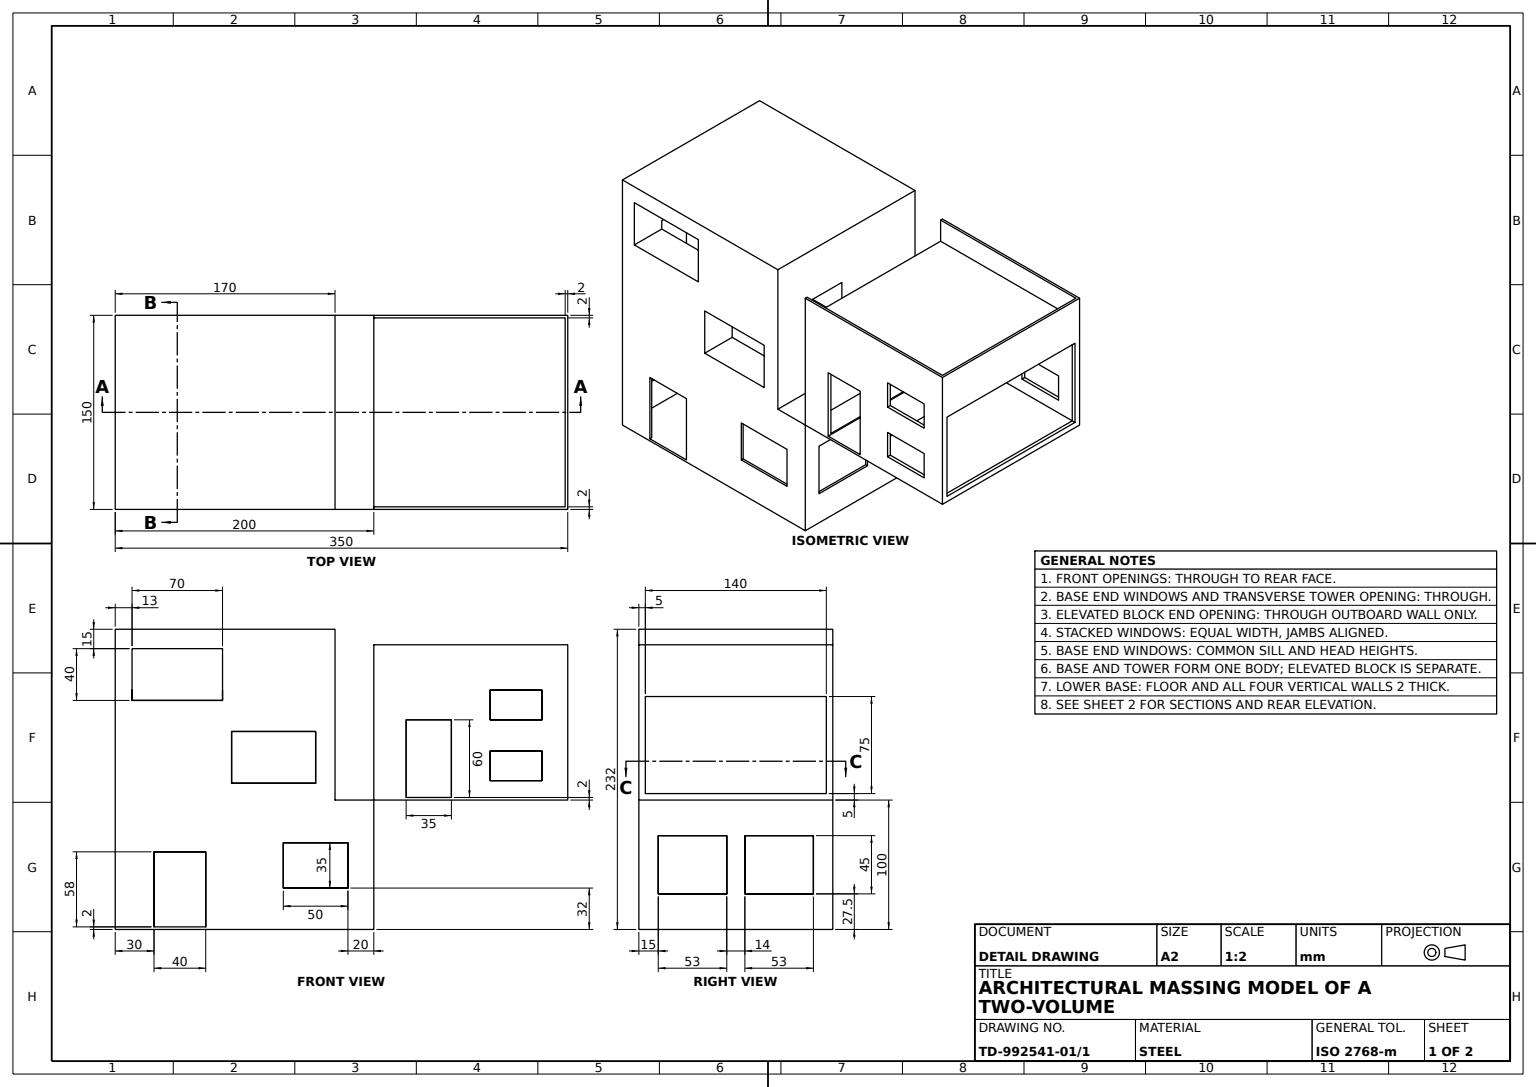
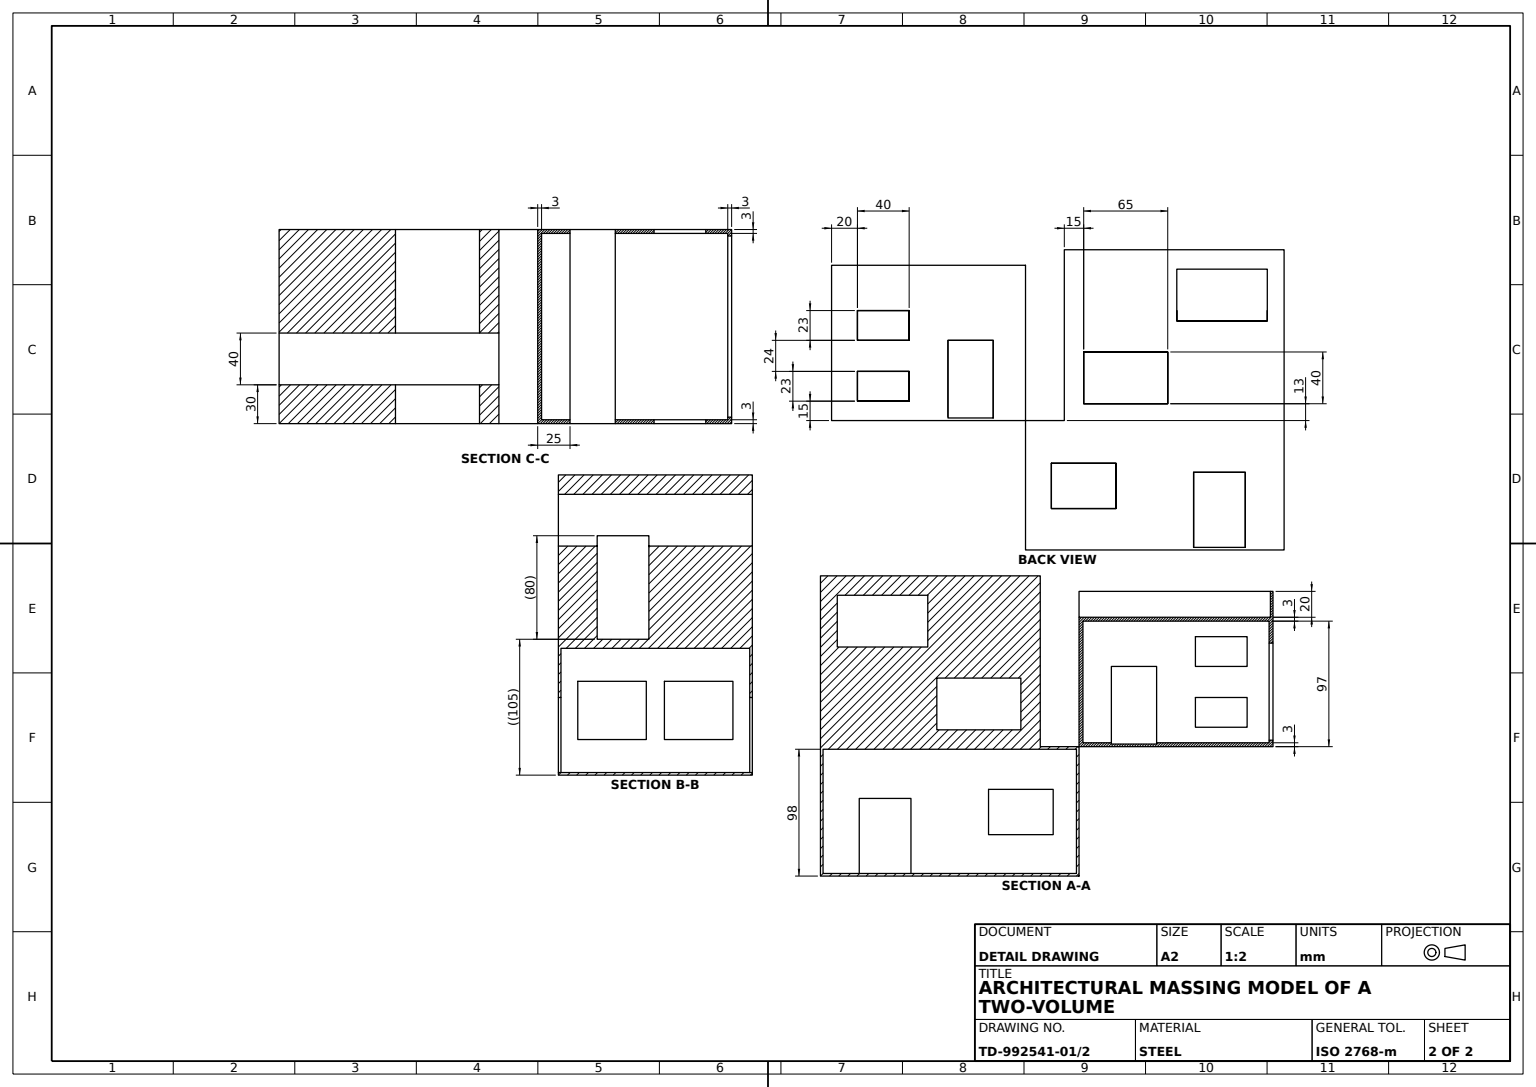
solid
v1 (330,115,-3)
v2 (330,115,0)
e1 v1 v2 LINE
v3 (330,138,0)
e2 v2 v3 LINE
v4 (330,138,-3)
e3 v4 v3 LINE
e4 v1 v4 LINE
face PLANE(AX(P(330,115,-213),D(1,0,0),D(0,0,-1))) rev [e1 e2 -e3 -e4]
v5 (200,220,-150)
v6 (350,220,-150)
e5 v5 v6 LINE
v7 (200,220,-148)
e6 v7 v5 LINE
v8 (348,220,-148)
e7 v7 v8 LINE
v9 (348,220,-2)
e8 v8 v9 LINE
v10 (200,220,-2)
e9 v9 v10 LINE
v11 (200,220,0)
e10 v10 v11 LINE
v12 (350,220,0)
e11 v12 v11 LINE
e12 v6 v12 LINE
face PLANE(AX(P(200,220,-2),D(0,1,0),D(0,0,1))) [-e5 -e6 e7 e8 e9 e10 -e11 -e12]
v13 (260,162,-150)
v14 (225,162,-150)
e13 v13 v14 LINE
v15 (260,162,-147)
e14 v13 v15 LINE
v16 (225,162,-147)
e15 v16 v15 LINE
e16 v14 v16 LINE
face PLANE(AX(P(225,162,-213),D(0,1,0),D(0,0,1))) rev [-e13 e14 -e15 -e16]
v17 (200,200,-148)
v18 (200,200,-2)
e17 v17 v18 LINE
v19 (348,200,-2)
e18 v18 v19 LINE
v20 (348,200,-148)
e19 v19 v20 LINE
e20 v20 v17 LINE
face PLANE(AX(P(0,200,0),D(0,-1,0),D(0,0,-1))) rev [e17 e18 e19 e20]
v21 (290,138,-3)
v22 (290,115,-3)
e21 v21 v22 LINE
v23 (290,138,0)
e22 v21 v23 LINE
v24 (290,115,0)
e23 v23 v24 LINE
e24 v22 v24 LINE
face PLANE(AX(P(290,115,-213),D(-1,0,0),D(0,0,1))) rev [-e21 e22 e23 -e24]
v25 (203,103,-3)
v26 (203,197,-3)
e25 v25 v26 LINE
v27 (203,103,-147)
e26 v27 v25 LINE
v28 (203,197,-147)
e27 v27 v28 LINE
e28 v26 v28 LINE
face PLANE(AX(P(203,103,-147),D(-1,0,0),D(0,0,1))) rev [-e25 -e26 e27 -e28]
v29 (290,162,-150)
v30 (330,162,-150)
e29 v29 v30 LINE
v31 (330,185,-150)
e30 v30 v31 LINE
v32 (290,185,-150)
e31 v31 v32 LINE
e32 v32 v29 LINE
v33 (350,100,-150)
e33 v6 v33 LINE
v34 (200,100,-150)
e34 v33 v34 LINE
e35 v5 v34 LINE
v35 (330,115,-150)
v36 (330,138,-150)
e36 v35 v36 LINE
v37 (290,138,-150)
e37 v36 v37 LINE
v38 (290,115,-150)
e38 v37 v38 LINE
e39 v38 v35 LINE
v39 (260,102,-150)
e40 v39 v13 LINE
v40 (225,102,-150)
e41 v14 v40 LINE
e42 v40 v39 LINE
face PLANE(AX(P(200,200,-150),D(0,0,1),D(1,0,0))) rev [e29 e30 e31 e32] [e5 e33 e34 -e35] [e36 e37 e38 e39] [e40 e13 e41 e42]
v41 (347,197,-147)
e43 v28 v41 LINE
v42 (347,197,-3)
e44 v41 v42 LINE
e45 v42 v26 LINE
face PLANE(AX(P(0,197,0),D(0,1,0),D(0,0,1))) rev [e28 e43 e44 e45]
v43 (290,185,-147)
e46 v32 v43 LINE
v44 (290,162,-147)
e47 v44 v43 LINE
e48 v29 v44 LINE
face PLANE(AX(P(290,162,-213),D(-1,0,0),D(0,0,1))) rev [e46 -e47 -e48 -e32]
v45 (347,103,-147)
v46 (260,103,-147)
e49 v45 v46 LINE
v47 (260,103,-3)
e50 v47 v46 LINE
v48 (347,103,-3)
e51 v47 v48 LINE
e52 v48 v45 LINE
face PLANE(AX(P(0,103,0),D(0,1,0),D(0,0,1))) [e49 -e50 e51 e52]
v49 (347,180,-145)
v50 (347,180,-5)
e53 v49 v50 LINE
v51 (350,180,-145)
e54 v49 v51 LINE
v52 (350,180,-5)
e55 v51 v52 LINE
e56 v50 v52 LINE
face PLANE(AX(P(237,180,-5),D(0,1,0),D(0,0,1))) rev [-e53 e54 e55 -e56]
v53 (290,138,-147)
e57 v37 v53 LINE
v54 (290,115,-147)
e58 v54 v53 LINE
e59 v38 v54 LINE
face PLANE(AX(P(290,115,-213),D(-1,0,0),D(0,0,1))) rev [e57 -e58 -e59 -e38]
v55 (350,105,-145)
e60 v55 v51 LINE
v56 (350,105,-5)
e61 v56 v55 LINE
e62 v52 v56 LINE
v57 (350,100,0)
e63 v12 v57 LINE
e64 v57 v33 LINE
face PLANE(AX(P(350,200,0),D(-1,0,0),D(0,0,1))) rev [-e55 -e60 -e61 -e62] [e12 e63 e64 -e33]
v58 (347,105,-5)
e65 v58 v56 LINE
e66 v50 v58 LINE
face PLANE(AX(P(237,105,-5),D(0,0,1),D(1,0,0))) rev [e56 e62 -e65 -e66]
e67 v4 v21 LINE
e68 v22 v1 LINE
v59 (225,103,-3)
e69 v25 v59 LINE
e70 v48 v42 LINE
v60 (260,162,-3)
e71 v47 v60 LINE
v61 (225,162,-3)
e72 v60 v61 LINE
e73 v61 v59 LINE
v62 (290,162,-3)
v63 (330,162,-3)
e74 v62 v63 LINE
v64 (330,185,-3)
e75 v63 v64 LINE
v65 (290,185,-3)
e76 v64 v65 LINE
e77 v65 v62 LINE
face PLANE(AX(P(203,103,-3),D(0,0,1),D(1,0,0))) rev [e4 e67 e21 e68] [-e69 e25 -e45 -e70 -e51 e71 e72 e73] [e74 e75 e76 e77]
v66 (347,105,-145)
e78 v66 v49 LINE
e79 v66 v55 LINE
face PLANE(AX(P(237,105,-145),D(0,0,-1),D(-1,0,0))) rev [-e54 -e78 e79 e60]
e80 v8 v20 LINE
e81 v17 v7 LINE
face PLANE(AX(P(0,0,-148),D(0,0,-1),D(-1,0,0))) rev [-e20 -e80 -e7 -e81]
e82 v3 v23 LINE
face PLANE(AX(P(290,138,-213),D(0,1,0),D(0,0,1))) rev [e3 e82 -e22 -e67]
v67 (330,138,-147)
e83 v36 v67 LINE
e84 v53 v67 LINE
face PLANE(AX(P(290,138,-213),D(0,1,0),D(0,0,1))) rev [-e37 e83 -e84 -e57]
e85 v58 v66 LINE
face PLANE(AX(P(237,105,-5),D(0,-1,0),D(0,0,-1))) rev [-e85 e65 e61 -e79]
v68 (330,185,-147)
e86 v31 v68 LINE
e87 v43 v68 LINE
face PLANE(AX(P(290,185,-213),D(0,1,0),D(0,0,1))) rev [e86 -e87 -e46 -e31]
v69 (225,162,0)
e88 v61 v69 LINE
v70 (225,102,0)
e89 v69 v70 LINE
e90 v40 v70 LINE
v71 (225,103,-147)
e91 v71 v16 LINE
e92 v71 v59 LINE
face PLANE(AX(P(225,102,-213),D(-1,0,0),D(0,0,1))) rev [e88 e89 -e90 -e41 e16 -e91 e92 -e73]
v72 (330,115,-147)
e93 v72 v54 LINE
e94 v35 v72 LINE
face PLANE(AX(P(290,115,-213),D(0,-1,0),D(0,0,-1))) rev [-e93 -e94 -e39 e59]
v73 (330,185,0)
e95 v64 v73 LINE
v74 (290,185,0)
e96 v73 v74 LINE
e97 v65 v74 LINE
face PLANE(AX(P(290,185,-213),D(0,1,0),D(0,0,1))) rev [e95 e96 -e97 -e76]
e98 v45 v41 LINE
e99 v71 v27 LINE
e100 v15 v46 LINE
v75 (330,162,-147)
e101 v68 v75 LINE
e102 v75 v44 LINE
e103 v67 v72 LINE
face PLANE(AX(P(203,103,-147),D(0,0,-1),D(-1,0,0))) rev [-e49 e98 -e43 -e27 -e99 e91 e15 e100] [e47 e87 e101 e102] [e58 e84 e103 e93]
e104 v30 v75 LINE
face PLANE(AX(P(290,162,-213),D(0,-1,0),D(0,0,-1))) rev [-e29 e48 -e102 -e104]
v76 (260,162,0)
e105 v60 v76 LINE
e106 v76 v69 LINE
face PLANE(AX(P(225,162,-213),D(0,1,0),D(0,0,1))) rev [-e72 e105 e106 -e88]
v77 (200,100,0)
e107 v77 v57 LINE
e108 v34 v77 LINE
face PLANE(AX(P(0,100,0),D(0,-1,0),D(0,0,-1))) [-e64 -e107 -e108 -e34]
v78 (290,162,0)
e109 v74 v78 LINE
e110 v62 v78 LINE
face PLANE(AX(P(290,162,-213),D(-1,0,0),D(0,0,1))) rev [-e77 e97 e109 -e110]
e111 v24 v2 LINE
face PLANE(AX(P(290,115,-213),D(0,-1,0),D(0,0,-1))) rev [-e68 e24 e111 -e1]
v79 (260,102,0)
e112 v39 v79 LINE
e113 v79 v76 LINE
face PLANE(AX(P(260,102,-213),D(1,0,0),D(0,0,-1))) rev [e112 e113 -e105 -e71 e50 -e100 -e14 -e40]
e114 v11 v77 LINE
v80 (330,162,0)
e115 v80 v73 LINE
e116 v78 v80 LINE
e117 v70 v79 LINE
face PLANE(AX(P(200,200,0),D(0,0,-1),D(-1,0,0))) rev [-e82 -e2 -e111 -e23] [e114 e107 -e63 e11] [-e109 -e96 -e115 -e116] [-e117 -e89 -e106 -e113]
e118 v9 v19 LINE
face PLANE(AX(P(348,0,0),D(-1,0,0),D(0,0,1))) [-e19 -e118 -e8 e80]
e119 v63 v80 LINE
face PLANE(AX(P(290,162,-213),D(0,-1,0),D(0,0,-1))) rev [e116 -e119 -e74 e110]
face PLANE(AX(P(330,162,-213),D(1,0,0),D(0,0,-1))) rev [-e86 -e30 e104 -e101]
face PLANE(AX(P(330,115,-213),D(1,0,0),D(0,0,-1))) rev [-e103 -e83 -e36 e94]
e120 v10 v18 LINE
face PLANE(AX(P(200,200,0),D(1,0,0),D(0,0,-1))) rev [e108 -e114 -e10 e120 -e17 e81 e6 e35]
face PLANE(AX(P(330,162,-213),D(1,0,0),D(0,0,-1))) rev [e115 -e95 -e75 e119]
face PLANE(AX(P(0,103,0),D(0,1,0),D(0,0,1))) [e26 e69 -e92 e99]
face PLANE(AX(P(0,0,-2),D(0,0,-1),D(-1,0,0))) [e118 -e18 -e120 -e9]
face PLANE(AX(P(225,102,-213),D(0,-1,0),D(0,0,-1))) rev [e90 e117 -e112 -e42]
face PLANE(AX(P(347,103,-147),D(1,0,0),D(0,0,-1))) rev [e66 e85 e78 e53] [-e44 -e98 -e52 e70]
solid
v81 (198,27.5,-15)
v82 (198,27.5,-68)
e121 v81 v82 LINE
v83 (198,72.5,-68)
e122 v82 v83 LINE
v84 (198,72.5,-15)
e123 v83 v84 LINE
e124 v84 v81 LINE
v85 (198,2,-148)
v86 (198,98,-148)
e125 v85 v86 LINE
v87 (198,2,-2)
e126 v87 v85 LINE
v88 (198,98,-2)
e127 v87 v88 LINE
e128 v86 v88 LINE
v89 (198,27.5,-82)
v90 (198,27.5,-135)
e129 v89 v90 LINE
v91 (198,72.5,-135)
e130 v90 v91 LINE
v92 (198,72.5,-82)
e131 v91 v92 LINE
e132 v92 v89 LINE
face PLANE(AX(P(198,2,-148),D(1,0,0),D(0,0,-1))) rev [e121 e122 e123 e124] [-e125 -e126 e127 -e128] [e129 e130 e131 e132]
v93 (0,27.5,-15)
v94 (0,27.5,-68)
e133 v93 v94 LINE
v95 (2,27.5,-15)
e134 v93 v95 LINE
v96 (2,27.5,-68)
e135 v96 v95 LINE
e136 v94 v96 LINE
face PLANE(AX(P(-132,27.5,-15),D(0,-1,0),D(0,0,-1))) rev [-e133 e134 -e135 -e136]
v97 (0,185,-70)
v98 (0,185,-30)
e137 v97 v98 LINE
v99 (13,185,-70)
e138 v97 v99 LINE
v100 (13,185,-30)
e139 v100 v99 LINE
e140 v98 v100 LINE
face PLANE(AX(P(-36,185,-30),D(0,1,0),D(0,0,1))) rev [-e137 e138 -e139 -e140]
v101 (200,27.5,-15)
v102 (200,27.5,-68)
e141 v101 v102 LINE
v103 (200,72.5,-15)
e142 v103 v101 LINE
v104 (200,72.5,-68)
e143 v104 v103 LINE
e144 v102 v104 LINE
v105 (200,0,0)
v106 (200,0,-150)
e145 v105 v106 LINE
v107 (200,100,-150)
e146 v107 v106 LINE
v108 (200,100,0)
e147 v108 v107 LINE
e148 v108 v105 LINE
v109 (200,27.5,-82)
v110 (200,27.5,-135)
e149 v109 v110 LINE
v111 (200,72.5,-82)
e150 v111 v109 LINE
v112 (200,72.5,-135)
e151 v112 v111 LINE
e152 v110 v112 LINE
face PLANE(AX(P(200,100,0),D(-1,0,0),D(0,0,1))) rev [-e141 -e142 -e143 -e144] [e145 -e146 -e147 e148] [-e149 -e150 -e151 -e152]
v113 (180,32,-150)
v114 (180,32,-148)
e153 v113 v114 LINE
v115 (130,32,-150)
e154 v115 v113 LINE
v116 (130,32,-148)
e155 v115 v116 LINE
e156 v114 v116 LINE
face PLANE(AX(P(130,32,-332),D(0,-1,0),D(0,0,-1))) rev [-e153 -e154 e155 -e156]
v117 (180,67,-150)
v118 (130,67,-150)
e157 v117 v118 LINE
v119 (180,67,-148)
e158 v117 v119 LINE
v120 (130,67,-148)
e159 v120 v119 LINE
e160 v118 v120 LINE
face PLANE(AX(P(130,67,-332),D(0,1,0),D(0,0,1))) rev [-e157 e158 -e159 -e160]
e161 v113 v117 LINE
e162 v118 v115 LINE
v121 (90,113,-150)
v122 (155,113,-150)
e163 v121 v122 LINE
v123 (155,153,-150)
e164 v122 v123 LINE
v124 (90,153,-150)
e165 v123 v124 LINE
e166 v124 v121 LINE
v125 (0,232,-150)
v126 (0,0,-150)
e167 v125 v126 LINE
v127 (170,232,-150)
e168 v127 v125 LINE
v128 (170,100,-150)
e169 v127 v128 LINE
e170 v107 v128 LINE
e171 v106 v126 LINE
v129 (30,60,-150)
v130 (30,2,-150)
e172 v129 v130 LINE
v131 (70,2,-150)
e173 v130 v131 LINE
v132 (70,60,-150)
e174 v131 v132 LINE
e175 v132 v129 LINE
v133 (13,177,-150)
v134 (83,177,-150)
e176 v133 v134 LINE
v135 (83,217,-150)
e177 v134 v135 LINE
v136 (13,217,-150)
e178 v135 v136 LINE
e179 v136 v133 LINE
face PLANE(AX(P(0,100,-150),D(0,0,1),D(1,0,0))) rev [e154 e161 e157 e162] [e163 e164 e165 e166] [-e167 -e168 e169 -e170 e146 e171] [e172 e173 e174 e175] [e176 e177 e178 e179]
v137 (90,153,-70)
e180 v124 v137 LINE
v138 (90,113,-70)
e181 v137 v138 LINE
e182 v121 v138 LINE
face PLANE(AX(P(90,113,-152),D(-1,0,0),D(0,0,1))) rev [e180 e181 -e182 -e166]
v139 (155,153,-70)
e183 v139 v137 LINE
e184 v123 v139 LINE
face PLANE(AX(P(155,153,-152),D(0,1,0),D(0,0,1))) rev [e183 -e180 -e165 e184]
v140 (130,32,-2)
v141 (180,32,-2)
e185 v140 v141 LINE
v142 (180,67,-2)
e186 v141 v142 LINE
v143 (130,67,-2)
e187 v142 v143 LINE
e188 v143 v140 LINE
v144 (2,2,-2)
v145 (2,98,-2)
e189 v144 v145 LINE
e190 v88 v145 LINE
v146 (70,2,-2)
e191 v146 v87 LINE
v147 (70,60,-2)
e192 v147 v146 LINE
v148 (30,60,-2)
e193 v148 v147 LINE
v149 (30,2,-2)
e194 v149 v148 LINE
e195 v144 v149 LINE
face PLANE(AX(P(2,2,-2),D(0,0,1),D(1,0,0))) rev [e185 e186 e187 e188] [e189 -e190 -e127 -e191 -e192 -e193 -e194 -e195]
v150 (170,100,0)
e196 v150 v108 LINE
e197 v150 v128 LINE
face PLANE(AX(P(0,100,0),D(0,-1,0),D(0,0,-1))) rev [e196 e147 e170 -e197]
v151 (0,72.5,-68)
v152 (0,72.5,-15)
e198 v151 v152 LINE
v153 (2,72.5,-68)
e199 v151 v153 LINE
v154 (2,72.5,-15)
e200 v154 v153 LINE
e201 v152 v154 LINE
face PLANE(AX(P(-132,72.5,-15),D(0,1,0),D(0,0,1))) rev [-e198 e199 -e200 -e201]
v155 (0,0,0)
e202 v126 v155 LINE
e203 v155 v105 LINE
face PLANE(AX(P(0,0,0),D(0,-1,0),D(0,0,-1))) [-e202 -e171 -e145 -e203]
v156 (0,27.5,-135)
v157 (2,27.5,-135)
e204 v156 v157 LINE
v158 (2,72.5,-135)
e205 v158 v157 LINE
v159 (0,72.5,-135)
e206 v159 v158 LINE
e207 v156 v159 LINE
face PLANE(AX(P(-132,27.5,-135),D(0,0,-1),D(-1,0,0))) rev [e204 -e205 -e206 -e207]
e208 v91 v112 LINE
e209 v92 v111 LINE
face PLANE(AX(P(-132,72.5,-82),D(0,1,0),D(0,0,1))) rev [e208 e151 -e209 -e131]
e210 v95 v154 LINE
e211 v153 v96 LINE
v160 (2,98,-148)
e212 v145 v160 LINE
v161 (2,2,-148)
e213 v161 v144 LINE
e214 v161 v160 LINE
v162 (2,27.5,-82)
e215 v157 v162 LINE
v163 (2,72.5,-82)
e216 v162 v163 LINE
e217 v163 v158 LINE
face PLANE(AX(P(2,2,-148),D(-1,0,0),D(0,0,1))) rev [e135 e210 e200 e211] [-e212 -e189 -e213 e214] [e205 e215 e216 e217]
v164 (83,217,0)
v165 (13,217,0)
e218 v164 v165 LINE
e219 v136 v165 LINE
e220 v135 v164 LINE
face PLANE(AX(P(13,217,-152),D(0,1,0),D(0,0,1))) rev [e218 -e219 -e178 e220]
v166 (155,153,-30)
v167 (155,153,0)
e221 v166 v167 LINE
v168 (155,113,-30)
e222 v166 v168 LINE
v169 (155,113,0)
e223 v168 v169 LINE
e224 v169 v167 LINE
face PLANE(AX(P(155,113,-152),D(1,0,0),D(0,0,-1))) rev [-e221 e222 e223 e224]
v170 (0,232,0)
e225 v125 v170 LINE
v171 (170,232,0)
e226 v170 v171 LINE
e227 v171 v127 LINE
face PLANE(AX(P(0,232,0),D(0,1,0),D(0,0,1))) [e225 e226 e227 e168]
v172 (30,2,-148)
e228 v172 v161 LINE
v173 (30,60,-148)
e229 v173 v172 LINE
v174 (70,60,-148)
e230 v174 v173 LINE
v175 (70,2,-148)
e231 v175 v174 LINE
e232 v85 v175 LINE
e233 v160 v86 LINE
e234 v116 v120 LINE
e235 v119 v114 LINE
face PLANE(AX(P(2,2,-148),D(0,0,-1),D(-1,0,0))) rev [-e214 -e228 -e229 -e230 -e231 -e232 e125 -e233] [e234 e159 e235 e156]
v176 (0,72.5,-82)
e236 v176 v163 LINE
e237 v159 v176 LINE
face PLANE(AX(P(-132,72.5,-82),D(0,1,0),D(0,0,1))) rev [-e217 -e236 -e237 e206]
e238 v83 v104 LINE
e239 v84 v103 LINE
face PLANE(AX(P(-132,72.5,-15),D(0,1,0),D(0,0,1))) rev [e238 e143 -e239 -e123]
v177 (83,185,-30)
v178 (83,177,-30)
e240 v177 v178 LINE
v179 (83,177,0)
e241 v178 v179 LINE
e242 v179 v164 LINE
v180 (83,177,-70)
e243 v134 v180 LINE
v181 (83,185,-70)
e244 v180 v181 LINE
e245 v181 v177 LINE
face PLANE(AX(P(83,217,-152),D(1,0,0),D(0,1,0))) rev [e240 e241 e242 -e220 -e177 e243 e244 e245]
v182 (130,32,0)
v183 (180,32,0)
e246 v182 v183 LINE
v184 (130,67,0)
e247 v184 v182 LINE
v185 (180,67,0)
e248 v185 v184 LINE
e249 v183 v185 LINE
v186 (30,60,0)
v187 (30,2,0)
e250 v186 v187 LINE
v188 (70,60,0)
e251 v188 v186 LINE
v189 (70,2,0)
e252 v189 v188 LINE
e253 v187 v189 LINE
v190 (90,113,0)
e254 v190 v169 LINE
v191 (90,153,0)
e255 v191 v190 LINE
e256 v167 v191 LINE
v192 (13,177,0)
e257 v165 v192 LINE
e258 v192 v179 LINE
e259 v171 v150 LINE
e260 v170 v155 LINE
face PLANE(AX(P(0,100,0),D(0,0,-1),D(-1,0,0))) rev [-e246 -e247 -e248 -e249] [-e250 -e251 -e252 -e253] [-e224 -e254 -e255 -e256] [-e257 -e218 -e242 -e258] [-e259 -e226 e260 e203 -e148 -e196]
face PLANE(AX(P(180,32,-332),D(1,0,0),D(0,0,-1))) rev [-e235 -e158 -e161 e153]
e261 v90 v110 LINE
e262 v89 v109 LINE
face PLANE(AX(P(-132,27.5,-82),D(0,-1,0),D(0,0,-1))) rev [-e261 -e129 e262 e149]
e263 v148 v186 LINE
e264 v149 v187 LINE
face PLANE(AX(P(30,2,-270),D(-1,0,0),D(0,0,1))) rev [e263 e250 -e264 e194]
v193 (0,27.5,-82)
e265 v193 v162 LINE
e266 v176 v193 LINE
face PLANE(AX(P(-132,27.5,-82),D(0,0,1),D(1,0,0))) rev [e236 -e216 -e265 -e266]
e267 v143 v184 LINE
e268 v142 v185 LINE
face PLANE(AX(P(130,67,-332),D(0,1,0),D(0,0,1))) rev [e248 -e267 -e187 e268]
v194 (170,185,-30)
v195 (170,105,-30)
e269 v194 v195 LINE
v196 (170,185,-70)
e270 v196 v194 LINE
v197 (170,105,-70)
e271 v197 v196 LINE
e272 v195 v197 LINE
face PLANE(AX(P(170,232,-150),D(-1,0,0),D(0,0,1))) rev [-e169 -e227 e259 e197] [-e269 -e270 -e271 -e272]
e273 v141 v183 LINE
face PLANE(AX(P(180,32,-332),D(1,0,0),D(0,0,-1))) rev [-e268 -e186 e273 e249]
v198 (0,105,-70)
e274 v198 v197 LINE
v199 (0,105,-30)
e275 v199 v198 LINE
e276 v199 v195 LINE
face PLANE(AX(P(-36,105,-30),D(0,-1,0),D(0,0,-1))) rev [-e274 -e275 e276 e272]
e277 v193 v156 LINE
face PLANE(AX(P(-132,27.5,-82),D(0,-1,0),D(0,0,-1))) rev [-e215 -e204 -e277 e265]
e278 v129 v173 LINE
e279 v130 v172 LINE
face PLANE(AX(P(30,2,-270),D(-1,0,0),D(0,0,1))) rev [-e172 e278 e229 -e279]
face PLANE(AX(P(-132,27.5,-82),D(0,0,1),D(1,0,0))) rev [-e132 e209 e150 -e262]
v200 (90,153,-30)
e280 v200 v166 LINE
v201 (90,113,-30)
e281 v201 v200 LINE
e282 v168 v201 LINE
e283 v177 v194 LINE
e284 v98 v199 LINE
v202 (13,177,-30)
e285 v202 v100 LINE
e286 v178 v202 LINE
face PLANE(AX(P(-36,105,-30),D(0,0,1),D(1,0,0))) rev [-e222 -e280 -e281 -e282] [-e240 e283 e269 -e276 -e284 e140 -e285 -e286]
e287 v147 v188 LINE
e288 v146 v189 LINE
face PLANE(AX(P(70,2,-270),D(1,0,0),D(0,0,-1))) rev [-e287 e192 e288 e252]
v203 (155,113,-70)
e289 v122 v203 LINE
e290 v203 v139 LINE
face PLANE(AX(P(155,113,-152),D(1,0,0),D(0,0,-1))) rev [-e184 -e164 e289 e290]
face PLANE(AX(P(-132,27.5,-135),D(0,0,-1),D(-1,0,0))) rev [-e130 e261 e152 -e208]
e291 v152 v93 LINE
face PLANE(AX(P(-132,27.5,-15),D(0,0,1),D(1,0,0))) rev [-e291 e201 -e210 -e134]
e292 v200 v191 LINE
e293 v201 v190 LINE
face PLANE(AX(P(90,113,-152),D(-1,0,0),D(0,0,1))) rev [e292 e255 -e293 e281]
face PLANE(AX(P(0,98,0),D(0,1,0),D(0,0,1))) rev [e212 e233 e128 e190]
face PLANE(AX(P(155,153,-152),D(0,1,0),D(0,0,1))) rev [e280 e221 e256 -e292]
face PLANE(AX(P(30,60,-270),D(0,1,0),D(0,0,1))) rev [e193 e287 e251 -e263]
e294 v202 v192 LINE
v204 (13,177,-70)
e295 v99 v204 LINE
e296 v133 v204 LINE
face PLANE(AX(P(13,217,-152),D(-1,0,0),D(0,-1,0))) rev [e257 -e294 e285 e139 e295 -e296 -e179 e219]
face PLANE(AX(P(13,177,-152),D(0,-1,0),D(0,0,-1))) rev [e258 -e241 e286 e294]
e297 v198 v97 LINE
e298 v181 v196 LINE
e299 v204 v180 LINE
e300 v138 v203 LINE
face PLANE(AX(P(-36,105,-70),D(0,0,-1),D(-1,0,0))) rev [-e138 -e297 e274 e271 -e298 -e244 -e299 -e295] [-e290 -e300 -e181 -e183]
face PLANE(AX(P(-36,185,-30),D(0,1,0),D(0,0,1))) rev [e270 -e283 -e245 e298]
e301 v82 v102 LINE
e302 v81 v101 LINE
face PLANE(AX(P(-132,27.5,-15),D(0,-1,0),D(0,0,-1))) rev [e141 -e301 -e121 e302]
face PLANE(AX(P(155,113,-152),D(0,-1,0),D(1,0,0))) rev [-e289 -e163 e182 e300]
e303 v94 v151 LINE
face PLANE(AX(P(0,100,0),D(1,0,0),D(0,0,-1))) rev [e207 e237 e266 e277] [e275 e297 e137 e284] [e198 e291 e133 e303] [e202 -e260 -e225 e167]
face PLANE(AX(P(130,32,-332),D(-1,0,0),D(0,0,1))) rev [e160 -e234 -e155 -e162]
e304 v140 v182 LINE
face PLANE(AX(P(130,32,-332),D(-1,0,0),D(0,0,1))) rev [-e188 e267 e247 -e304]
face PLANE(AX(P(13,177,-152),D(0,-1,0),D(0,0,-1))) rev [e299 -e243 -e176 e296]
face PLANE(AX(P(155,113,-152),D(0,-1,0),D(1,0,0))) rev [e254 -e223 e282 e293]
e305 v132 v174 LINE
face PLANE(AX(P(30,60,-270),D(0,1,0),D(0,0,1))) rev [e305 e230 -e278 -e175]
face PLANE(AX(P(-132,27.5,-68),D(0,0,-1),D(-1,0,0))) rev [e136 -e211 -e199 -e303]
face PLANE(AX(P(-132,27.5,-68),D(0,0,-1),D(-1,0,0))) rev [e144 -e238 -e122 e301]
face PLANE(AX(P(-132,27.5,-15),D(0,0,1),D(1,0,0))) rev [e142 -e302 -e124 e239]
e306 v131 v175 LINE
face PLANE(AX(P(30,2,-270),D(0,-1,0),D(0,0,-1))) rev [e213 e195 e264 e253 -e288 e191 e126 e232 -e306 -e173 e279 e228]
face PLANE(AX(P(130,32,-332),D(0,-1,0),D(0,0,-1))) rev [-e185 e304 e246 -e273]
face PLANE(AX(P(70,2,-270),D(1,0,0),D(0,0,-1))) rev [e231 -e305 -e174 e306]
